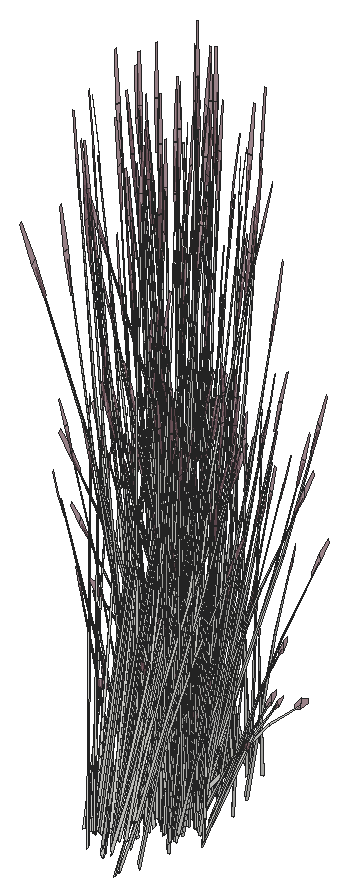
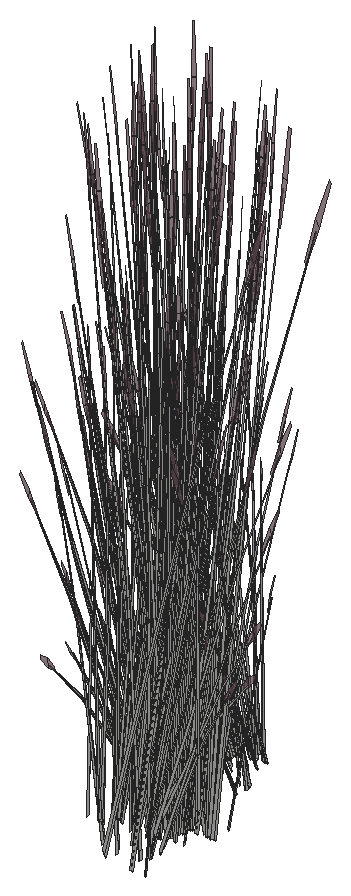
# SketchUp Ruby script. Lengths in inches.
U = 1.inch
M = Sketchup.active_model
def pt(a) = Geom::Point3d.new(a.map { |v| v * U })
def face(e, loops, mat)
  f = e.add_face(loops[0].map { |a| pt(a) })
  loops[1..].each { |l| e.add_face(l.map { |a| pt(a) }).erase! }
  f.material = f.back_material = mat if mat
  f
end
# faces: each face lists its corners as indices into pts; further lists are holes
def faces(e, pts, list, mat = nil) = list.each { |f| face(e, (f[0].is_a?(Array) ? f : [f]).map { |l| l.map { |i| pts[i] } }, mat) }
# xy, xz, yz: faces in a plane at the given z, y or x. An outline is a flat list of corners, or four numbers for a rectangle; further outlines are holes
def ring(l) = l.size == 4 ? [[l[0], l[1]], [l[2], l[1]], [l[2], l[3]], [l[0], l[3]]] : l.each_slice(2).to_a
def flat(e, list, mat, &to3) = list.each { |f| face(e, (f[0].is_a?(Array) ? f : [f]).map { |l| ring(l).map { |u, v| to3.(u, v) } }, mat) }
def xy(e, z, list, mat = nil) = flat(e, list, mat) { |x, y| [x, y, z] }
def xz(e, y, list, mat = nil) = flat(e, list, mat) { |x, z| [x, y, z] }
def yz(e, x, list, mat = nil) = flat(e, list, mat) { |y, z| [x, y, z] }
def lines(e, pts, list) = list.each { |a, b| e.add_line(pt(pts[a]), pt(pts[b])) }
# prism: a flat outline (further loops are holes) pulled along v
def prism(e, loops, v, mat = nil)
  f = face(e, loops, mat); d = Geom::Vector3d.new(v.map { |x| x * U })
  f.pushpull(f.normal.samedirection?(d) ? d.length : -d.length)
end
def box(e, o, s, mat = nil) = prism(e, [[o, [o[0] + s[0], o[1], o[2]], [o[0] + s[0], o[1] + s[1], o[2]], [o[0], o[1] + s[1], o[2]]]], [0, 0, s[2]], mat)
def at(x, y, z, deg = 0) = Geom::Transformation.translation(pt([x, y, z])) * Geom::Transformation.rotation(ORIGIN, Z_AXIS, deg.degrees)
def axes(o, x, y, z) = Geom::Transformation.new([*x, 0, *y, 0, *z, 0, *pt(o).to_a, 1])
def part(name) = M.definitions.add(name)
# library, detail: a bought-in or finely detailed component or shape, given as its bounding box
def library(name, o, s) = part(name).tap { |d| box(d.entities, o, s) }
def detail(e, o, s) = box(e.add_group.entities, o, s)
def put(e, d, t, mat = nil) = e.add_instance(d, t).tap { |i| i.material = mat if mat }
def group(e, t, mat = nil) = e.add_group.tap { |g| g.transformation = t; g.material = mat if mat }.entities
root = M.entities
M.materials.add("LightPink_Translucent").color = [144, 107, 117]
M.materials["LightPink_Translucent"].alpha = 0.75
c1 = part("blade")
p = [[2.15,0.21,22],[0,0.17,0],[0.09,0.45,0],[2.18,0.31,22],[2.29,0.31,22],[0.38,0.45,0],
  [2.48,0.24,33],[2.49,0.24,33],[2.48,0.22,33]]
faces(c1.entities,p,[[0,1,2,3],[4,5,2,3],[6,3,4,7],[8,0,3,6]])
c2 = part("seeds")
p = [[0.3,-0.1,1.38],[-0.01,-0.03,1.59],[-0.01,-0.03,0.03],[0.14,-0.07,-0.07],[0.29,-0.03,3],[0.15,0.01,3.11]]
faces(c2.entities,p,[[0,1,2,3],[1,0,4,5]],"LightPink_Translucent")
c3 = part("blade with seeds")
put(c3.entities,c1,at(0,0,0))
put(c3.entities,c2,axes([2.4,0.25,30.99],[1.5799,-0.05474,1.17369],[-0.12525,1.92788,0.29478],[-0.07173,-0.02425,1.56792]))
put(root,c3,axes([410.64,282.69,-7.6],[-0.42027,-0.02533,0.05988],[0.01152,-0.38243,0.47138],[-0.04398,0.14649,0.71878]))
put(root,c3,axes([410.77,282.73,-7.59],[-0.36417,-0.37086,0.447],[0.38674,-0.31985,0.36857],[-0.06718,0.174,0.92496]))
put(root,c3,axes([413.32,282.83,-7.64],[0.50465,-0.12921,-0.47583],[0.08828,0.48932,-0.36857],[0.13555,0.14022,0.91046]))
put(root,c3,axes([410.1875,287.81,-7.6],[0.23243,-0.34529,0.05988],[0.331,0.20103,0.47138],[-0.10701,-0.1107,0.71878]))
put(root,c3,axes([411.92,282.9,-7.3],[0.15418,-0.41799,0.32977],[0.44981,0.12192,-0.42575],[0.04124,0.16829,0.81462]))
put(root,c3,axes([410.11,289.73,-10.05],[-0.21003,-0.55738,-0.65031],[0.60499,-0.20074,-0.17068],[-0.02321,-0.18874,1.43544]))
put(root,c3,axes([412.92,288.02,-10.61],[-0.07655,-0.04282,1.6421],[-0.19662,-0.47839,-0.25086],[0.13264,-0.12982,0.2797]))
put(root,c3,axes([414.02,283.33,-9.52],[-0.32795,-0.01705,0.97832],[0.21658,-0.36206,0.54015],[0.12956,0.12863,0.76741]))
put(root,c3,axes([411.34,288.13,-7.3],[-0.15418,0.41799,0.32977],[-0.44981,-0.12192,-0.42575],[-0.04124,-0.16829,0.81462]))
put(root,c3,axes([413.08,283.23,-7.6],[-0.23243,0.34529,0.05988],[-0.331,-0.20103,0.47138],[0.10701,0.1107,0.71878]))
put(root,c3,axes([412.49,288.31,-7.59],[0.36417,0.37086,0.447],[-0.38674,0.31985,0.36857],[0.06718,-0.174,0.92496]))
put(root,c3,axes([412.53,284.39,-6.74],[0.35341,-0.31182,-0.06041],[0.32382,0.34152,-0.27392],[0.0228,0.09677,0.90349]))
put(root,c3,axes([412.62,288.34,-7.6],[0.42027,0.02533,0.05988],[-0.01152,0.38243,0.47138],[0.04398,-0.14649,0.71878]))
put(root,c3,axes([413.17,283.13,-7.59],[-0.50866,0.12474,0.447],[-0.08828,-0.48932,0.36857],[0.11963,0.14421,0.92496]))
put(root,c3,axes([412.31,288.6,-7.3],[-0.34603,0.28618,0.32977],[-0.32756,-0.32677,-0.42575],[0.04984,-0.16603,0.81462]))
put(root,c3,axes([410.66,281.79,-8.39],[0.09522,-0.18683,1.59586],[0.39947,0.38663,0.12904],[-0.18021,0.24097,0.68222]))
put(root,c3,axes([412.92,289.375,-7.36],[0.26714,-0.42887,-0.66157],[0.46811,0.30479,0.07984],[0.1595,-0.15539,0.93586]))
put(root,c3,axes([410.03,288.125,-9.79],[-0.31974,-0.54466,0],[0.53494,-0.30375,-0.48057],[0.12184,-0.06918,1.52448]))
put(root,c3,axes([412.91,289.17,-7.64],[-0.13138,-0.49631,-0.47583],[0.49754,-0.08682,-0.36857],[0.14258,-0.13331,0.91046]))
put(root,c3,axes([412.95,282.45,-9.59],[0.00902,-0.18018,1.33163],[0.43127,-0.20126,-0.28638],[0.13313,0.21566,0.56934]))
put(root,c3,axes([410.73,287.47,-10.02],[-0.35341,0.31182,-0.03625],[-0.32382,-0.34152,-0.16435],[-0.0228,-0.09677,0.54209]))
put(root,c3,axes([411.79,283.28,-7.6],[-0.37684,0.18473,0.05988],[-0.18445,-0.33686,0.47138],[0.03639,0.14849,0.71878]))
put(root,c3,axes([410.77,282.84,-7.78],[-0.34603,0.28618,-0.32977],[-0.32756,-0.32677,0.42575],[-0.04984,0.16603,0.81462]))
put(root,c3,axes([409.58,282.75,-7.61],[-0.01271,0.10756,1.62908],[0.36076,0.37419,-0.25764],[-0.09444,0.17695,0.13065]))
put(root,c3,axes([410.73,282.51,-6.97],[0.56206,0.02693,-0.12569],[-0.01536,0.50991,-0.69765],[-0.03904,0.19638,1.06006]))
put(root,c3,axes([411.77,283.08,-7.3125],[0.50045,-0.25306,-0.11324],[0.24593,0.44915,-0.62851],[0.06603,0.18927,0.95501]))
put(root,c3,axes([411.92,283.25,-7.28],[-0.50393,-0.1421,0.49617],[0.17232,-0.46717,0.40911],[0.03028,0.18372,1.0267]))
put(root,c3,axes([413.14,289.53,-7.3125],[-0.47307,-0.29971,-0.11324],[0.27254,-0.43404,-0.62851],[0.13365,-0.15087,0.95501]))
put(root,c3,axes([410.99,283.95,-9.42],[-0.01324,-0.32319,1.06958],[0.33072,0.23052,0.78586],[-0.06504,0.15405,0.23558]))
put(root,c3,axes([411.86,283.18,-10.61],[0.08277,-0.02958,1.6421],[0.49786,0.16279,-0.25086],[0.01456,0.18348,0.2797]))
put(root,c3,axes([411.1875,291.16,-8.9],[0.44194,0.21918,1.40854],[-0.43295,0.47219,0.557],[-0.19393,-0.27986,1.18082]))
put(root,c3,axes([410.26,288.2,-7.3],[0.07899,0.43781,0.32977],[-0.45153,0.11561,-0.42575],[-0.12128,-0.12546,0.81462]))
put(root,c3,axes([408.875,289.65,-10.12],[0,-0.54355,-0.46235],[0.57217,0,0],[0,-0.1238,1.46668]))
put(root,c3,axes([410.47,288.04,-10.12],[0.47863,-0.27177,-0.46235],[0.28609,0.48733,0],[0.10901,-0.0619,1.46668]))
put(root,c3,axes([413.31,288.98,-9.59],[-0.1827,-0.0161,1.33163],[-0.18717,-0.43188,-0.28638],[0.22444,-0.12218,0.56934]))
put(root,c3,axes([411.12,282.7,-7.34],[0.3661,0.36521,-0.52818],[-0.38674,0.31985,-0.40911],[-0.0557,0.18556,1.01061]))
put(root,c3,axes([414.3,289.4,-7.62],[-0.0668,-0.00413,1.65179],[-0.27738,-0.44233,-0.15608],[0.11139,-0.14544,0.29231]))
put(root,c3,axes([410.72,283.25,-9.37],[0.46459,-0.09625,0.0606],[0.10681,0.38778,-0.80367],[-0.02945,0.1963,0.72038]))
put(root,c3,axes([412.2,283.06,-7.64],[0.50273,0.13626,-0.47583],[-0.17232,0.46717,-0.36857],[0.0461,0.18809,0.91046]))
put(root,c3,axes([412.49,282.09,-8.39],[-0.1169,-0.17452,1.59586],[0.54019,-0.14692,0.12904],[0.12209,0.27397,0.68222]))
put(root,c3,axes([411.03,289.16,-10.08],[0.34446,-0.40855,-0.58063],[0.42791,0.37046,-0.15239],[0.13803,-0.10191,1.28164]))
put(root,c3,axes([413.52,288.1875,-9.42],[-0.17034,0.27669,1.06958],[-0.14642,-0.37174,0.78586],[0.14069,-0.09315,0.23558]))
put(root,c3,axes([411.97,283.34,-7.78],[-0.15418,0.41799,-0.32977],[-0.44981,-0.12192,0.42575],[0.04124,0.16829,0.81462]))
put(root,c3,axes([413.27,289.23,-7.78],[0.44516,-0.07768,-0.32977],[0.11755,0.44407,0.42575],[0.12757,-0.11927,0.81462]))
put(root,c3,axes([411,282.54,-7.03],[-0.01331,0.50278,-0.73435],[-0.56035,-0.03377,0.08862],[-0.05914,0.213,1.03881]))
put(root,c3,axes([409.54,283.86,-7.62],[0.05802,-0.03282,1.65179],[0.47954,0.21828,-0.15608],[-0.01127,0.18175,0.29231]))
put(root,c3,axes([410.43,289.87,-9.94],[0.24813,-0.48978,-0.41661],[0.51557,0.23571,0.2005],[0,-0.1129,1.33761]))
put(root,c3,axes([410.66,289.63,-9.52],[-0.05959,-0.62022,-0.27094],[0.62068,-0.0375,-0.46562],[0.1093,-0.08261,1.4872]))
put(root,c3,axes([409.12,289.66,-10.11],[0.35699,-0.33913,-0.28847],[0.35699,0.33913,0.28847],[0,-0.10923,1.29413]))
put(root,c3,axes([411.53,282.18,-8.39],[-0.01252,-0.20862,1.59586],[0.54251,0.1384,0.12904],[-0.03356,0.2973,0.68222]))
put(root,c3,axes([408.98,288.04,-10.02],[-0.14753,0.44383,-0.03625],[-0.45406,-0.13653,-0.16435],[-0.06894,-0.07259,0.54209]))
put(root,c3,axes([412.91,289.49,-7.3],[-0.44516,0.07768,0.32977],[-0.11755,-0.44407,-0.42575],[0.12757,-0.11927,0.81462]))
put(root,c3,axes([410.37,290.28,-9.52],[-0.57594,-0.25935,-0.27094],[0.27732,-0.5474,-0.46562],[-0.0181,-0.1344,1.4872]))
put(root,c3,axes([408.73,290.0625,-9.79],[-0.63949,0,0],[0,-0.60749,-0.48057],[0,-0.13836,1.52448]))
put(root,c3,axes([412.02,282.97,-7.36],[0.24409,0.44196,-0.66157],[-0.50245,0.2463,0.07984],[0.05708,0.21354,0.93586]))
put(root,c3,axes([410.58,288.26,-10.11],[0.47712,0.13449,-0.28847],[-0.12013,0.47362,0.28847],[0.09619,-0.05462,1.29413]))
put(root,c3,axes([410.61,283.66,-9.59],[0.16138,-0.08575,1.33163],[0.39845,0.25854,-0.28638],[-0.1186,0.22371,0.56934]))
put(root,c3,axes([411.66,284.08,-7.61],[0.06483,0.08753,1.62908],[0.52315,0.03439,-0.25764],[0.05261,0.19303,0.13065]))
put(root,c3,axes([413.3125,289.42,-7.6],[0.35109,0.22859,0.05988],[-0.2044,0.32553,0.47138],[0.11256,-0.10524,0.71878]))
put(root,c3,axes([413.21,289.32,-7.59],[0.12683,0.50025,0.447],[-0.49754,0.08682,0.36857],[0.14663,-0.11765,0.92496]))
put(root,c3,axes([414.56,289.93,-7.61],[0.07097,-0.08279,1.62908],[-0.09083,-0.50786,-0.25764],[0.17806,-0.09629,0.13065]))
put(root,c3,axes([409.23,289.9,-9.83],[-0.47569,0.45698,0.2864],[-0.47598,-0.45217,-0.33981],[-0.01661,-0.12977,1.53541]))
put(root,c3,axes([410.82,283.24,-8.87],[0.01124,-0.2806,1.43727],[0.50537,0.14821,0.19862],[-0.04379,0.29905,0.67868]))
put(root,c3,axes([410.74,290.11,-9.73],[0.57623,0.26344,0.22409],[-0.27732,0.5474,0.46562],[0,-0.12618,1.49497]))
put(root,c3,axes([410.52,290.85,-9.73],[0.13555,-0.64407,-0.21817],[0.64269,0.11227,0.47743],[-0.1123,-0.08895,1.45677]))
put(root,c3,axes([410.55,289.75,-9.47],[-0.55535,0.03355,0.41661],[-0.05022,-0.55698,-0.2005],[0.09942,-0.05645,1.33761]))
put(root,c3,axes([409.12,290.15,-9.69],[0,0.54355,0.46235],[-0.57217,0,0],[0,-0.1238,1.46668]))
put(root,c3,axes([413.16,290.7,-7.3125],[-0.25732,-0.49218,-0.11324],[0.45669,-0.24187,-0.62851],[0.19245,-0.06494,0.95501]))
put(root,c3,axes([413.14,290.28,-7.64],[0.13855,-0.49442,-0.47583],[0.47502,0.16947,-0.36857],[0.19125,-0.04534,0.91046]))
put(root,c3,axes([412.39,288.26,-9.79],[0.31974,-0.54466,0],[0.53494,0.30375,-0.48057],[0.12184,0.06918,1.52448]))
put(root,c3,axes([410.47,290.59,-9.94],[-0.30722,-0.45622,-0.41661],[0.46535,-0.32126,0.2005],[-0.09942,-0.05645,1.33761]))
put(root,c3,axes([410.54,289.95,-9.8],[0.22235,0.6078,0.42607],[-0.63531,0.21135,0.16719],[0.00776,-0.11168,1.47927]))
put(root,c3,axes([413.64,290.41,-10.15],[-0.32938,0.06523,1.31842],[-0.05243,-0.51922,0.07547],[0.2307,-0.07859,0.75023]))
put(root,c3,axes([414.24,289.95,-9.89],[-0.31706,-0.34757,-0.06041],[0.34725,-0.31847,-0.27392],[0.09839,-0.02242,0.90349]))
put(root,c3,axes([410.42,290.43,-9.47],[-0.24813,0.48978,0.41661],[-0.51557,-0.23571,-0.2005],[0,-0.1129,1.33761]))
put(root,c3,axes([411.33,290,-9.95],[0,-0.62892,0],[0.63949,0,0],[0,0,1.6711]))
put(root,c3,axes([412.11,288.55,-9.69],[-0.47863,-0.27177,0.46235],[0.28609,-0.48733,0],[0.10901,0.0619,1.46668]))
put(root,c3,axes([413.05,290.46,-7.36],[0.44939,-0.24006,-0.66157],[0.25044,0.49415,0.07984],[0.21713,-0.05613,0.93586]))
put(root,c3,axes([411.03,289.6,-9.8],[-0.42403,0.49328,0.42607],[-0.50377,-0.43543,0.16719],[0.10223,-0.04923,1.47927]))
put(root,c3,axes([411.49,290.49,-9.86],[-0.47569,-0.46784,-0.05709],[0.47598,-0.46812,0],[-0.01661,-0.01634,1.63492]))
put(root,c3,axes([410.3,288.79,-9.7],[-0.14774,0.54019,0.16428],[-0.54062,-0.15287,0.32672],[0.09339,-0.00263,1.49371]))
put(root,c3,axes([412.98,290.55,-7.3],[-0.42502,-0.15163,0.32977],[0.12396,-0.44238,-0.42575],[0.17112,-0.04056,0.81462]))
put(root,c3,axes([410.07,289.23,-10.52],[-0.50338,0.21762,1.20058],[-0.16022,-0.62439,0.4665],[0.30911,0.01039,1.36553]))
put(root,c3,axes([411.42,289.39,-9.5625],[0.09866,-0.48509,0.13483],[0.48202,0.0842,-0.38503],[0.08772,0.04981,1.18024]))
put(root,c3,axes([410.59,290.54,-9.8],[0.64638,0.11452,0.42607],[-0.13155,0.64678,0.16719],[-0.09446,-0.06245,1.47927]))
put(root,c3,axes([414,290.08,-10.61],[-0.02673,-0.08252,1.6421],[0.18538,-0.48271,-0.25086],[0.187,-0.00694,0.2797]))
put(root,c3,axes([410.04,294.48,-8.39],[0.1169,0.17452,1.59586],[-0.54019,0.14692,0.12904],[-0.12209,-0.27397,0.68222]))
put(root,c3,axes([411.22,289.52,-9.47],[-0.30722,-0.45622,0.41661],[0.46535,-0.32126,-0.2005],[0.09942,0.05645,1.33761]))
put(root,c3,axes([409.63,291.61,-10.11],[-0.12013,-0.47362,-0.28847],[0.47712,-0.13449,0.28847],[-0.09619,-0.05462,1.29413]))
put(root,c3,axes([410.94,293.33,-7.61],[-0.07822,-0.07621,1.62908],[-0.52201,0.04832,-0.25764],[-0.08331,-0.18228,0.13065]))
put(root,c3,axes([412.15,294.23,-9.59],[-0.14537,0.11002,1.33163],[-0.43536,-0.19256,-0.28638],[0.0807,-0.23948,0.56934]))
put(root,c3,axes([411.48,294.61,-7.36],[-0.24409,-0.44196,-0.66157],[0.50245,-0.2463,0.07984],[-0.05708,-0.21354,0.93586]))
put(root,c3,axes([410.24,291.58,-9.7],[0.54955,-0.14427,0.16428],[0.1357,0.53689,0.32672],[-0.04901,-0.07823,1.49371]))
put(root,c3,axes([411.375,289.55,-9.52],[0.51635,-0.36087,-0.27094],[0.34336,0.5099,-0.46562],[0.1274,0.05178,1.4872]))
put(root,c3,axes([413.43,290.5,-7.78],[0.42502,0.15163,-0.32977],[-0.12396,0.44238,0.42575],[0.17112,-0.04056,0.81462]))
put(root,c3,axes([409.9,294.02,-9.59],[-0.03097,0.17781,1.33163],[-0.45273,0.14885,-0.28638],[-0.10583,-0.22982,0.56934]))
put(root,c3,axes([412.68,288.59,-10.12],[0.47863,0.27177,-0.46235],[-0.28609,0.48733,0],[0.10901,0.0619,1.46668]))
put(root,c3,axes([411.77,290.14,-9.95],[0.57217,0,0],[0,0.56272,0],[0,0,1.66132]))
put(root,c3,axes([411.0625,293.63,-10.61],[-0.08578,0.01958,1.6421],[-0.47437,-0.22044,-0.25086],[0.00796,-0.18387,0.2797]))
put(root,c3,axes([410.8,290.85,-9.52],[-0.51635,0.36087,-0.27094],[-0.34336,-0.5099,-0.46562],[-0.1274,-0.05178,1.4872]))
put(root,c3,axes([411.93,288.82,-9.7],[-0.54955,0.14427,0.16428],[-0.1357,-0.53689,0.32672],[0.04901,0.07823,1.49371]))
put(root,c3,axes([412.27,289.95,-8.39],[-0.21212,0.01231,1.59586],[0.14072,-0.53355,0.12904],[0.3023,0.033,0.68222]))
put(root,c3,axes([412.5,295.04,-7.36],[0.01331,-0.50278,-0.66157],[0.56035,0.03377,0.07984],[0.05914,-0.213,0.93586]))
put(root,c3,axes([412.54,288.79,-10.11],[0.12013,0.47362,-0.28847],[-0.47712,0.13449,0.28847],[0.09619,0.05462,1.29413]))
put(root,c3,axes([413.28,294.26,-7.61],[-0.00494,-0.10818,1.62908],[-0.41695,-0.31265,-0.25764],[0.06446,-0.18952,0.13065]))
put(root,c3,axes([413.37,290.6875,-7.6],[0.18783,0.37061,0.05988],[-0.34252,0.1814,0.47138],[0.15099,-0.03579,0.71878]))
put(root,c3,axes([411.53,294.24,-7.78],[0.15418,-0.41799,-0.32977],[0.44981,0.12192,0.42575],[-0.04124,-0.16829,0.81462]))
put(root,c3,axes([411.87,294.79,-8.39],[-0.09522,0.18683,1.59586],[-0.39947,-0.38663,0.12904],[0.18021,-0.24097,0.68222]))
put(root,c3,axes([413.17,293.87,-7.62],[-0.05194,0.04152,1.65179],[-0.50886,-0.14007,-0.15608],[-0.01842,-0.18118,0.29231]))
put(root,c3,axes([411.58,289.85,-9.78],[-0.64638,-0.11452,0.45814],[0.13155,-0.64678,0.17978],[0.09446,0.06245,1.59061]))
put(root,c3,axes([413.33,290.56,-7.59],[-0.14449,0.4956,0.447],[-0.47502,-0.16947,0.36857],[0.1868,-0.02978,0.92496]))
put(root,c3,axes([411.07,291.45,-9.95],[-0.16686,-0.46861,0],[0.47648,-0.16411,0],[0,0,1.4375]))
put(root,c3,axes([410.75,291.01,-9.5625],[-0.09866,0.48509,0.13483],[-0.48202,-0.0842,-0.38503],[-0.08772,-0.04981,1.18024]))
put(root,c3,axes([411.3,294.52,-7.64],[-0.50273,-0.13626,-0.47583],[0.17232,-0.46717,-0.36857],[-0.0461,-0.18809,0.91046]))
put(root,c3,axes([411.61,293.35,-9.42],[0.06561,0.31695,1.06958],[-0.36394,-0.17555,0.78586],[0.03916,-0.16229,0.23558]))
put(root,c3,axes([411.69,291.39,-9.97],[0.53691,-0.18442,-0.17877],[0.18866,0.53125,0.00007],[0.05927,-0.02038,1.61933]))
put(root,c3,axes([411.88,291.61,-9.7],[0.14774,-0.54019,0.16428],[0.54062,0.15287,0.32672],[-0.09339,0.00263,1.49371]))
put(root,c3,axes([412.39,294.88,-7.64],[-0.3661,-0.36521,-0.47583],[0.38674,-0.31985,-0.36857],[0.0557,-0.18556,0.91046]))
put(root,c3,axes([411.76,290.38,-9.9375],[0.35699,0.35109,0],[-0.35699,0.35109,0],[0,0,1.57621]))
put(root,c3,axes([410.4,293.08,-7.62],[-0.00954,0.06515,1.65179],[-0.47055,0.23645,-0.15608],[-0.13847,-0.12087,0.29231]))
put(root,c3,axes([412.72,290.23,-9.7],[-0.40181,-0.39593,0.16428],[0.40492,-0.38402,0.32672],[-0.04438,0.08086,1.49371]))
put(root,c3,axes([411.98,289.63,-10.08],[0.53199,0.08911,-0.58063],[-0.11226,0.54969,-0.15239],[0.15876,0.06661,1.28164]))
put(root,c3,axes([414.33,290.59,-9.42],[-0.31598,0.08973,1.06958],[0.14873,-0.37085,0.78586],[0.16763,0.02538,0.23558]))
put(root,c3,axes([410.95,291.66,-9.95],[-0.51557,-0.24403,0],[0.24813,-0.50705,0],[0,0,1.51513]))
put(root,c3,axes([411.38,291.01,-9.7],[-0.49938,-0.43748,-0.23459],[0.42021,-0.49126,0.51337],[-0.13447,0.05118,1.56642]))
put(root,c3,axes([410.3,294.23,-7.26],[0.56969,-0.13971,0.50064],[0.09887,0.54803,0.4128],[-0.13398,-0.16152,1.03595]))
put(root,c3,axes([410.06,291.85,-9.69],[0.47863,0.27177,0.46235],[-0.28609,0.48733,0],[-0.10901,-0.0619,1.46668]))
put(root,c3,axes([411.58,294.33,-7.59],[0.50393,0.1421,0.447],[-0.17232,0.46717,0.36857],[-0.03028,-0.18372,0.92496]))
put(root,c3,axes([411.73,294.5,-7.3125],[-0.50045,0.25306,-0.11324],[-0.24593,-0.44915,-0.62851],[-0.06603,-0.18927,0.95501]))
put(root,c3,axes([411.75,289.97,-9.47],[0.24813,-0.48978,0.41661],[0.51557,0.23571,-0.2005],[0,0.1129,1.33761]))
put(root,c3,axes([412.77,295.07,-7.3125],[-0.56206,-0.02693,-0.11324],[0.01536,-0.50991,-0.62851],[0.03904,-0.19638,0.95501]))
put(root,c3,axes([412.73,294.74,-7.78],[0.34603,-0.28618,-0.32977],[0.32756,0.32677,0.42575],[0.04984,-0.16603,0.81462]))
put(root,c3,axes([414.18,292.16,-7.62],[-0.04624,-0.04758,1.65179],[0.10116,-0.51007,-0.15608],[0.18215,-0.03259,0.29231]))
put(root,c3,axes([409.74,293.73,-9.42],[0.26677,0.18918,1.06958],[-0.38851,0.11372,0.78586],[-0.08313,-0.14539,0.23558]))
put(root,c3,axes([411.72,294.3,-7.6],[0.37684,-0.18473,0.05988],[0.18445,0.33686,0.47138],[-0.03639,-0.14849,0.71878]))
put(root,c3,axes([410.23,294.39,-7.78],[-0.07899,-0.43781,-0.32977],[0.45153,-0.11561,0.42575],[-0.12128,-0.12546,0.81462]))
put(root,c3,axes([411.66,290.25,-9.87],[0,0.62861,-0.05249],[-0.63949,0,0],[0,0.01975,1.67027]))
put(root,c3,axes([411.7,289.81,-9.94],[0.30722,0.45622,-0.41661],[-0.46535,0.32126,0.2005],[0.09942,0.05645,1.33761]))
put(root,c3,axes([413.78,291.73,-8.34],[-0.09788,-0.45691,-0.03251],[0.46264,-0.10504,-0.14742],[0.09661,0.02897,0.48626]))
put(root,c3,axes([412.58,291.72,-7.3125],[0.02738,-0.55277,-0.11324],[0.51847,0.01511,-0.62851],[0.19968,0.0384,0.95501]))
put(root,c3,axes([413.05,290.24,-9.69],[0,-0.54355,0.46235],[0.57217,0,0],[0,0.1238,1.46668]))
put(root,c3,axes([411.62,290.65,-9.47],[0.55535,-0.03355,0.41661],[0.05022,0.55698,-0.2005],[-0.09942,0.05645,1.33761]))
put(root,c3,axes([411.97,290.08,-9.5625],[0.47648,-0.15851,0.13483],[0.16686,0.45265,-0.38503],[0,0.09962,1.18024]))
put(root,c3,axes([412.5,291.5,-7.3],[-0.29098,-0.34031,0.32977],[0.33226,-0.32215,-0.42575],[0.16881,0.04902,0.81462]))
put(root,c3,axes([411.125,290.92,-9.94],[-0.55535,0.03355,-0.41661],[-0.05022,-0.55698,0.2005],[-0.09942,0.05645,1.33761]))
put(root,c3,axes([410.43,294.35,-7.6],[0.23243,-0.34529,0.05988],[0.331,0.20103,0.47138],[-0.10701,-0.1107,0.71878]))
put(root,c3,axes([413.74,291.1875,-9.59],[-0.12317,-0.13368,1.33163],[0.16025,-0.44223,-0.28638],[0.24919,0.05991,0.56934]))
put(root,c3,axes([410.35,296.27,-10.05],[-0.21003,-0.55738,-0.65031],[0.60499,-0.20074,-0.17068],[-0.02321,-0.18874,1.43544]))
put(root,c3,axes([413.16,294.57,-10.61],[-0.07655,-0.04282,1.6421],[-0.19662,-0.47839,-0.25086],[0.13264,-0.12982,0.2797]))
put(root,c3,axes([411.54,291.67,-9.95],[0.51557,0.24403,0],[-0.24813,0.50705,0],[0,0,1.62917]))
put(root,c3,axes([411.58,294.68,-7.3],[-0.15418,0.41799,0.32977],[-0.44981,-0.12192,-0.42575],[-0.04124,-0.16829,0.81462]))
put(root,c3,axes([413.03,291.39,-7.61],[0.10971,-0.00919,1.62908],[0.30091,-0.42228,-0.25764],[0.19514,0.05574,0.13065]))
put(root,c3,axes([411.74,292.21,-9.96],[-0.31576,-0.54657,-0.04789],[0.53494,-0.30375,0.48057],[-0.13182,0.05204,1.52373]))
put(root,c3,axes([412.73,294.85,-7.59],[0.36417,0.37086,0.447],[-0.38674,0.31985,0.36857],[0.06718,-0.174,0.92496]))
put(root,c3,axes([411.63,290.89,-9.5625],[0.37783,0.32657,0.13483],[-0.31516,0.36844,-0.38503],[-0.08772,0.04981,1.18024]))
put(root,c3,axes([412.86,294.89,-7.6],[0.42027,0.02533,0.05988],[-0.01152,0.38243,0.47138],[0.04398,-0.14649,0.71878]))
put(root,c3,axes([412.55,295.15,-7.3],[-0.34603,0.28618,0.32977],[-0.32756,-0.32677,-0.42575],[0.04984,-0.16603,0.81462]))
put(root,c3,axes([413.16,295.92,-7.36],[0.26714,-0.42887,-0.66157],[0.46811,0.30479,0.07984],[0.1595,-0.15539,0.93586]))
put(root,c3,axes([410.27,294.67,-9.79],[-0.31974,-0.54466,0],[0.53494,-0.30375,-0.48057],[0.12184,-0.06918,1.52448]))
put(root,c3,axes([413.15,295.72,-7.64],[-0.13138,-0.49631,-0.47583],[0.49754,-0.08682,-0.36857],[0.14258,-0.13331,0.91046]))
put(root,c3,axes([412.61,291.45,-7.36],[0.51122,0.01309,-0.66157],[-0.03434,0.5511,0.07984],[0.21658,0.05816,0.93586]))
put(root,c3,axes([410.97,294.01,-10.02],[-0.35341,0.31182,-0.03625],[-0.32382,-0.34152,-0.16435],[-0.0228,-0.09677,0.54209]))
put(root,c3,axes([412.03,291.9,-9.69],[0.47863,-0.27177,0.46235],[0.28609,0.48733,0],[-0.10901,0.0619,1.46668]))
put(root,c3,axes([411.35,291.47,-9.87],[0.22235,0.62444,-0.05599],[-0.63531,0.21881,0],[0.00776,0.02181,1.60327]))
put(root,c3,axes([413.38,296.07,-7.3125],[-0.47307,-0.29971,-0.11324],[0.27254,-0.43404,-0.62851],[0.13365,-0.15087,0.95501]))
put(root,c3,axes([411.6,292.14,-10.11],[-0.47712,-0.13449,-0.28847],[0.12013,-0.47362,0.28847],[-0.09619,0.05462,1.29413]))
put(root,c3,axes([408.95,290.81,-7.3],[0.44516,-0.07768,0.32977],[0.11755,0.44407,-0.42575],[-0.12757,0.11927,0.81462]))
put(root,c3,axes([413.44,290.34,-9.79],[0.63949,0,0],[0,0.60749,-0.48057],[0,0.13836,1.52448]))
put(root,c3,axes([413.1875,290.65,-9.95],[-0.63917,-0.00435,-0.04634],[0,-0.60749,0.46507],[-0.02009,0.13829,1.47457]))
put(root,c3,axes([411.8,290.12,-9.52],[0.57594,0.25935,-0.27094],[-0.27732,0.5474,-0.46562],[0.0181,0.1344,1.4872]))
put(root,c3,axes([411.43,297.71,-8.9],[0.44194,0.21918,1.40854],[-0.43295,0.47219,0.557],[-0.19393,-0.27986,1.18082]))
put(root,c3,axes([412.91,291.68,-7.78],[0.29098,0.34031,-0.32977],[-0.33226,0.32215,0.42575],[0.16881,0.04902,0.81462]))
put(root,c3,axes([410.5,294.75,-7.3],[0.07899,0.43781,0.32977],[-0.45153,0.11561,-0.42575],[-0.12128,-0.12546,0.81462]))
put(root,c3,axes([413.05,290.74,-10.11],[-0.35699,0.33913,-0.28847],[-0.35699,-0.33913,0.28847],[0,0.10923,1.29413]))
put(root,c3,axes([411.52,290.77,-9.52],[0.05959,0.62022,-0.27094],[-0.62068,0.0375,-0.46562],[-0.1093,0.08261,1.4872]))
put(root,c3,axes([409.12,296.19,-10.12],[0,-0.54355,-0.46235],[0.57217,0,0],[0,-0.1238,1.46668]))
put(root,c3,axes([410.71,294.59,-10.12],[0.47863,-0.27177,-0.46235],[0.28609,0.48733,0],[0.10901,-0.0619,1.46668]))
put(root,c3,axes([412.77,291.8125,-7.6],[-0.02575,0.41332,0.05988],[-0.38885,-0.01133,0.47138],[0.14895,0.04325,0.71878]))
put(root,c3,axes([413.55,295.52,-9.59],[-0.1827,-0.0161,1.33163],[-0.18717,-0.43188,-0.28638],[0.22444,-0.12218,0.56934]))
put(root,c3,axes([414.55,295.94,-7.62],[-0.0668,-0.00413,1.65179],[-0.27738,-0.44233,-0.15608],[0.11139,-0.14544,0.29231]))
